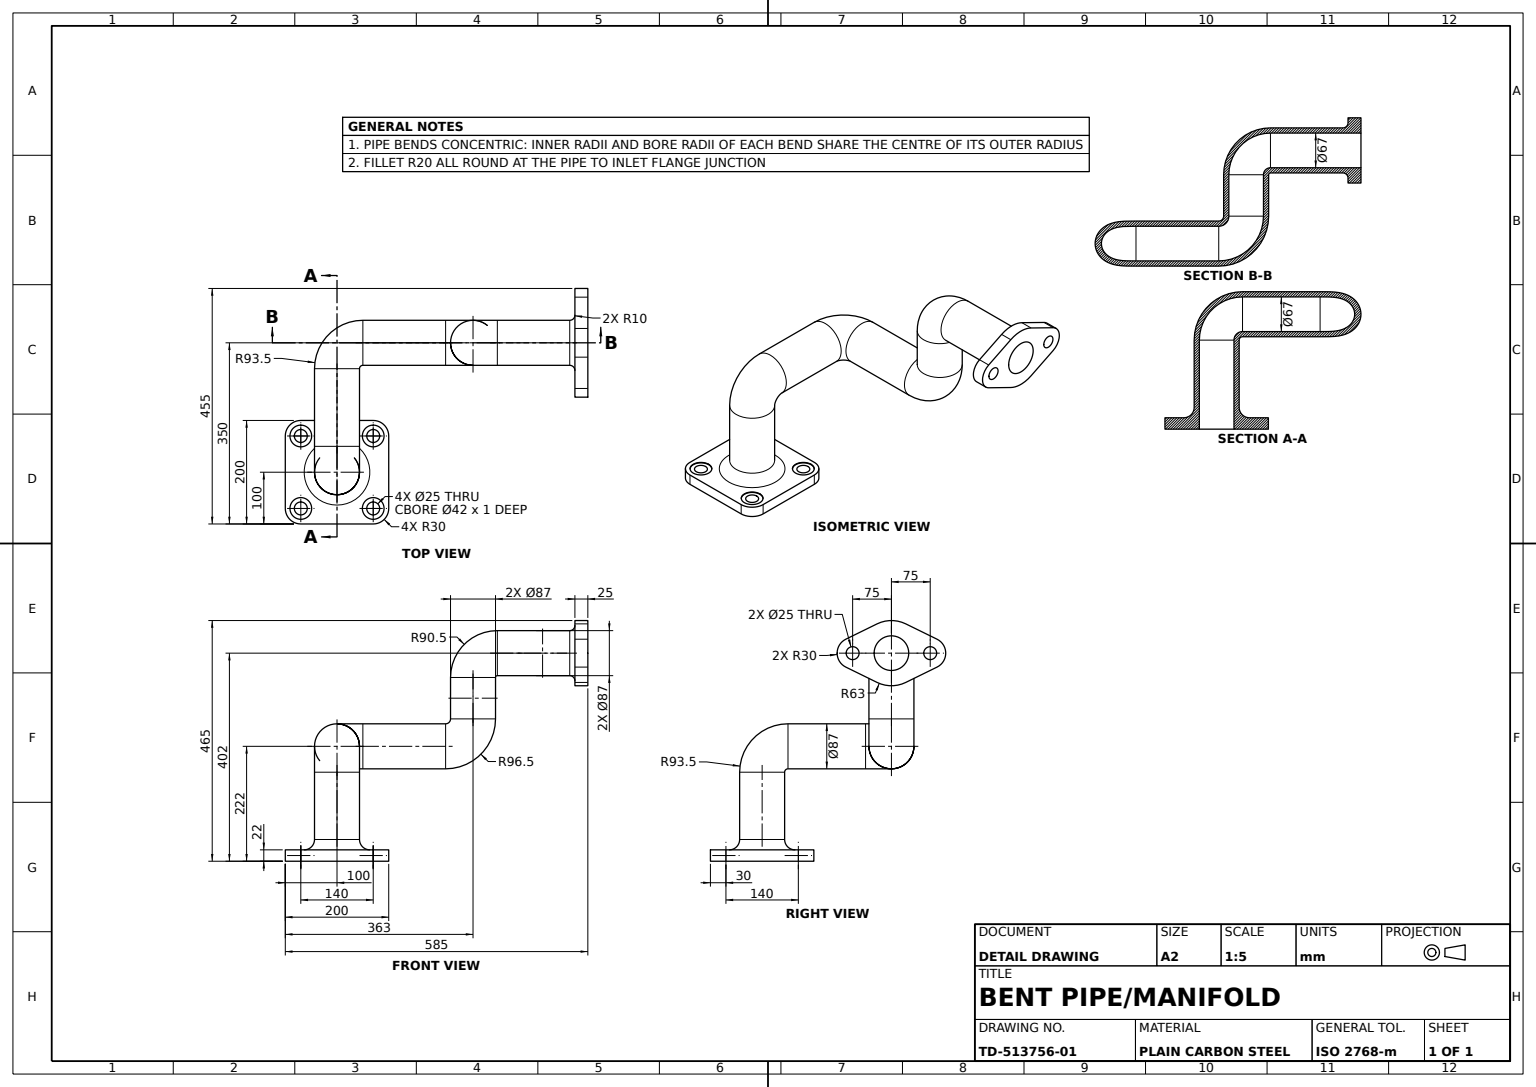
solid
v1 (70,21,-49)
v2 (70,21,-91)
e1 v1 v2 CIRCLE(AX(P(70,21,-70),D(0,1,0),D(0,0,1)),21)
e2 v2 v1 CIRCLE(AX(P(70,21,-70),D(0,1,0),D(0,0,1)),21)
v3 (70,21,-82.5)
v4 (70,21,-57.5)
e3 v3 v4 CIRCLE(AX(P(70,21,-70),D(0,1,0),D(0,0,1)),12.5)
e4 v4 v3 CIRCLE(AX(P(70,21,-70),D(0,1,0),D(0,0,1)),12.5)
face PLANE(AX(P(70,21,-70),D(0,1,0),D(0,0,1))) [e1 e2] [-e3 -e4]
v5 (485,458.57386,-277.72)
v6 (460,458.57386,-277.72)
e5 v5 v6 LINE
v7 (460,458.57386,-222.28)
e6 v6 v7 CIRCLE(AX(P(460,402,-250),D(1,0,0),D(0,0,-1)),63)
v8 (485,458.57386,-222.28)
e7 v8 v7 LINE
e8 v5 v8 CIRCLE(AX(P(485,402,-250),D(1,0,0),D(0,0,-1)),63)
face CYL(AX(P(485,402,-250),D(-1,0,0),D(0,0,1)),63) [e5 e6 -e7 -e8]
v9 (263,275,-216.5)
v10 (263,355,-216.5)
e9 v9 v10 LINE
v11 (296.5,355,-250)
e10 v10 v11 CIRCLE(AX(P(263,355,-250),D(0,1,0),D(0,0,-1)),33.5)
v12 (263,355,-283.5)
e11 v11 v12 CIRCLE(AX(P(263,355,-250),D(0,1,0),D(0,0,-1)),33.5)
v13 (263,275,-283.5)
e12 v13 v12 LINE
v14 (296.5,275,-250)
e13 v14 v13 CIRCLE(AX(P(263,275,-250),D(0,1,0),D(0,0,-1)),33.5)
e14 v9 v14 CIRCLE(AX(P(263,275,-250),D(0,1,0),D(0,0,-1)),33.5)
face CYL(AX(P(263,275,-250),D(0,1,0),D(0,0,1)),33.5) rev [e9 e10 e11 -e12 -e13 -e14]
v15 (50,222,-293.5)
v16 (50,222,-206.5)
e15 v15 v16 CIRCLE(AX(P(50,222,-250),D(1,0,0),D(0,0,-1)),43.5)
v17 (210,222,-206.5)
e16 v16 v17 LINE
v18 (210,265.5,-250)
e17 v18 v17 CIRCLE(AX(P(210,222,-250),D(1,0,0),D(0,-1,0)),43.5)
v19 (210,222,-293.5)
e18 v19 v18 CIRCLE(AX(P(210,222,-250),D(1,0,0),D(0,-1,0)),43.5)
e19 v15 v19 LINE
face CYL(AX(P(50,222,-250),D(1,0,0),D(0,0,-1)),43.5) [e15 e16 -e17 -e18 -e19]
v20 (0,42,-43.5)
v21 (0,172,-43.5)
e20 v20 v21 LINE
v22 (0,172,43.5)
e21 v22 v21 CIRCLE(AX(P(0,172,0),D(0,1,0),D(0,0,-1)),43.5)
v23 (0,42,43.5)
e22 v23 v22 LINE
e23 v23 v20 CIRCLE(AX(P(0,42,0),D(0,1,0),D(0,0,1)),43.5)
face CYL(AX(P(0,22,0),D(0,1,0),D(0,0,1)),43.5) [e20 -e21 -e22 e23]
v24 (0,0,-33.5)
v25 (0,172,-33.5)
e24 v24 v25 LINE
v26 (0,0,33.5)
e25 v26 v24 CIRCLE(AX(P(0,0,0),D(0,1,0),D(0,0,1)),33.5)
v27 (0,172,33.5)
e26 v26 v27 LINE
e27 v27 v25 CIRCLE(AX(P(0,172,0),D(0,1,0),D(0,0,1)),33.5)
face CYL(AX(P(0,-3,0),D(0,1,0),D(0,0,1)),33.5) rev [-e24 -e25 e26 e27]
v28 (70,0,-57.5)
e28 v4 v28 LINE
v29 (70,0,-82.5)
e29 v29 v28 CIRCLE(AX(P(70,0,-70),D(0,1,0),D(0,0,1)),12.5)
e30 v3 v29 LINE
face CYL(AX(P(70,22,-70),D(0,-1,0),D(0,0,-1)),12.5) rev [e3 e28 -e29 -e30]
v30 (43.5,222,-50)
v31 (43.5,222,-200)
e31 v30 v31 LINE
v32 (0,178.5,-50)
e32 v30 v32 CIRCLE(AX(P(0,222,-50),D(0,0,-1),D(-1,0,0)),43.5)
v33 (-43.5,222,-50)
e33 v32 v33 CIRCLE(AX(P(0,222,-50),D(0,0,-1),D(-1,0,0)),43.5)
v34 (-43.5,222,-200)
e34 v33 v34 LINE
e35 v31 v34 CIRCLE(AX(P(0,222,-200),D(0,0,-1),D(1,0,0)),43.5)
face CYL(AX(P(0,222,-50),D(0,0,-1),D(-1,0,0)),43.5) [-e31 e32 e33 e34 -e35]
v35 (485,402,-283.5)
v36 (485,402,-216.5)
e36 v35 v36 CIRCLE(AX(P(485,402,-250),D(1,0,0),D(0,0,-1)),33.5)
v37 (310,402,-216.5)
e37 v37 v36 LINE
v38 (310,435.5,-250)
e38 v38 v37 CIRCLE(AX(P(310,402,-250),D(1,0,0),D(0,0,-1)),33.5)
v39 (310,402,-283.5)
e39 v39 v38 CIRCLE(AX(P(310,402,-250),D(1,0,0),D(0,0,-1)),33.5)
e40 v39 v35 LINE
face CYL(AX(P(310,402,-250),D(1,0,0),D(0,0,-1)),33.5) rev [e36 -e37 -e38 -e39 e40]
v40 (100,22,-70)
v41 (100,0,-70)
e41 v40 v41 LINE
v42 (70,0,-100)
e42 v41 v42 CIRCLE(AX(P(70,0,-70),D(0,1,0),D(0,0,-1)),30)
v43 (70,22,-100)
e43 v43 v42 LINE
e44 v40 v43 CIRCLE(AX(P(70,22,-70),D(0,1,0),D(0,0,-1)),30)
face CYL(AX(P(70,22,-70),D(0,-1,0),D(0,0,-1)),30) [e41 e42 -e43 -e44]
v44 (70,21,49)
v45 (70,22,49)
e45 v44 v45 LINE
v46 (70,22,91)
e46 v45 v46 CIRCLE(AX(P(70,22,70),D(0,1,0),D(0,0,1)),21)
v47 (70,21,91)
e47 v47 v46 LINE
e48 v44 v47 CIRCLE(AX(P(70,21,70),D(0,1,0),D(0,0,1)),21)
face CYL(AX(P(70,21,70),D(0,1,0),D(0,0,1)),21) rev [e45 e46 -e47 -e48]
v48 (70,22,-49)
e49 v1 v48 LINE
v49 (70,22,-91)
e50 v48 v49 CIRCLE(AX(P(70,22,-70),D(0,1,0),D(0,0,1)),21)
e51 v2 v49 LINE
face CYL(AX(P(70,21,-70),D(0,1,0),D(0,0,1)),21) rev [-e1 e49 e50 -e51]
v50 (229.5,275,-250)
e52 v50 v9 CIRCLE(AX(P(263,275,-250),D(0,1,0),D(0,0,-1)),33.5)
v51 (210,188.5,-250)
e53 v51 v14 CIRCLE(AX(P(210,275,-250),D(0,0,1),D(1,0,0)),86.5)
v52 (210,222,-216.5)
e54 v52 v51 CIRCLE(AX(P(210,222,-250),D(1,0,0),D(0,0,-1)),33.5)
v53 (210,255.5,-250)
e55 v53 v52 CIRCLE(AX(P(210,222,-250),D(1,0,0),D(0,0,-1)),33.5)
e56 v53 v50 CIRCLE(AX(P(210,275,-250),D(0,0,1),D(1,0,0)),19.5)
face TORUS(AX(P(210,275,-250),D(0,0,1),D(1,0,0)),53,33.5) rev [e52 e14 -e53 -e54 -e55 e56]
v54 (485,345.42614,-277.72)
v55 (460,345.42614,-277.72)
e57 v54 v55 LINE
v56 (460,375.060067,-338.2)
e58 v55 v56 LINE
v57 (485,375.060067,-338.2)
e59 v57 v56 LINE
e60 v54 v57 LINE
face PLANE(AX(P(485,345.42614,-277.72),D(0,0.897997773,0.44),D(0,-0.44,0.897997773))) rev [e57 e58 -e59 -e60]
e61 v24 v26 CIRCLE(AX(P(0,0,0),D(0,1,0),D(0,0,1)),33.5)
e62 v25 v27 CIRCLE(AX(P(0,172,0),D(0,1,0),D(0,0,1)),33.5)
face CYL(AX(P(0,-3,0),D(0,1,0),D(0,0,1)),33.5) rev [-e61 e24 e62 -e26]
v58 (70,0,82.5)
v59 (70,0,57.5)
e63 v58 v59 CIRCLE(AX(P(70,0,70),D(0,1,0),D(0,0,1)),12.5)
v60 (70,21,82.5)
e64 v60 v58 LINE
v61 (70,21,57.5)
e65 v60 v61 CIRCLE(AX(P(70,21,70),D(0,1,0),D(0,0,1)),12.5)
e66 v61 v59 LINE
face CYL(AX(P(70,22,70),D(0,-1,0),D(0,0,-1)),12.5) rev [-e63 -e64 e65 e66]
e67 v34 v15 CIRCLE(AX(P(50,222,-200),D(0,-1,0),D(0,0,-1)),93.5)
e68 v34 v31 CIRCLE(AX(P(0,222,-200),D(0,0,-1),D(1,0,0)),43.5)
e69 v31 v16 CIRCLE(AX(P(50,222,-200),D(0,-1,0),D(0,0,-1)),6.5)
face TORUS(AX(P(50,222,-200),D(0,-1,0),D(0,0,-1)),50,43.5) [-e67 e68 e69 -e15]
v62 (-70,21,57.5)
v63 (-70,21,82.5)
e70 v62 v63 CIRCLE(AX(P(-70,21,70),D(0,1,0),D(0,0,1)),12.5)
e71 v63 v62 CIRCLE(AX(P(-70,21,70),D(0,1,0),D(0,0,1)),12.5)
v64 (-70,21,49)
v65 (-70,21,91)
e72 v64 v65 CIRCLE(AX(P(-70,21,70),D(0,1,0),D(0,0,1)),21)
e73 v65 v64 CIRCLE(AX(P(-70,21,70),D(0,1,0),D(0,0,1)),21)
face PLANE(AX(P(-70,21,70),D(0,1,0),D(0,0,1))) [-e70 -e71] [e72 e73]
v66 (0,22,63.5)
e74 v23 v66 CIRCLE(AX(P(0,42,63.5),D(-1,0,0),D(0,0,1)),20)
e75 v20 v23 CIRCLE(AX(P(0,42,0),D(0,1,0),D(0,0,1)),43.5)
v67 (0,22,-63.5)
e76 v20 v67 CIRCLE(AX(P(0,42,-63.5),D(1,0,0),D(0,0,-1)),20)
e77 v66 v67 CIRCLE(AX(P(0,22,0),D(0,-1,0),D(0,0,1)),63.5)
face TORUS(AX(P(0,42,0),D(0,1,0),D(0,0,1)),63.5,20) rev [-e74 -e75 e76 -e77]
v68 (-70,0,82.5)
e78 v63 v68 LINE
v69 (-70,0,57.5)
e79 v62 v69 LINE
e80 v68 v69 CIRCLE(AX(P(-70,0,70),D(0,1,0),D(0,0,1)),12.5)
face CYL(AX(P(-70,22,70),D(0,-1,0),D(0,0,-1)),12.5) rev [-e78 e71 e79 -e80]
v70 (460,428.939933,-338.2)
e81 v56 v70 CIRCLE(AX(P(460,402,-325),D(1,0,0),D(0,0,-1)),30)
v71 (485,428.939933,-338.2)
e82 v71 v70 LINE
e83 v57 v71 CIRCLE(AX(P(485,402,-325),D(1,0,0),D(0,0,-1)),30)
face CYL(AX(P(485,402,-325),D(-1,0,0),D(0,0,1)),30) [e59 e81 -e82 -e83]
v72 (485,375.060067,-161.8)
v73 (460,375.060067,-161.8)
e84 v72 v73 LINE
v74 (460,345.42614,-222.28)
e85 v73 v74 LINE
v75 (485,345.42614,-222.28)
e86 v75 v74 LINE
e87 v72 v75 LINE
face PLANE(AX(P(485,375.060067,-161.8),D(0,0.897997773,-0.44),D(0,0.44,0.897997773))) rev [e84 e85 -e86 -e87]
v76 (-70,0,100)
v77 (70,0,100)
e88 v76 v77 LINE
v78 (70,22,100)
e89 v78 v77 LINE
v79 (-70,22,100)
e90 v79 v78 LINE
e91 v79 v76 LINE
face PLANE(AX(P(-70,22,100),D(0,0,-1),D(-1,0,0))) rev [e88 -e89 -e90 e91]
e92 v16 v15 CIRCLE(AX(P(50,222,-250),D(1,0,0),D(0,0,-1)),43.5)
face TORUS(AX(P(50,222,-200),D(0,-1,0),D(0,0,-1)),50,43.5) [-e69 e35 e67 -e92]
v80 (485,402,-337.5)
v81 (460,402,-337.5)
e93 v80 v81 LINE
v82 (460,402,-312.5)
e94 v82 v81 CIRCLE(AX(P(460,402,-325),D(1,0,0),D(0,0,-1)),12.5)
v83 (485,402,-312.5)
e95 v83 v82 LINE
e96 v83 v80 CIRCLE(AX(P(485,402,-325),D(1,0,0),D(0,0,-1)),12.5)
face CYL(AX(P(485,402,-325),D(-1,0,0),D(0,0,1)),12.5) rev [e93 -e94 -e95 e96]
v84 (0,265.5,-50)
e97 v84 v30 CIRCLE(AX(P(0,222,-50),D(0,0,-1),D(-1,0,0)),43.5)
e98 v22 v84 CIRCLE(AX(P(0,172,-50),D(-1,0,0),D(0,0,1)),93.5)
e99 v21 v32 CIRCLE(AX(P(0,172,-50),D(-1,0,0),D(0,0,1)),6.5)
face TORUS(AX(P(0,172,-50),D(-1,0,0),D(0,0,1)),50,43.5) [-e32 -e97 -e98 e21 e99]
v85 (0,255.5,-50)
e100 v27 v85 CIRCLE(AX(P(0,172,-50),D(-1,0,0),D(0,0,1)),83.5)
v86 (0,188.5,-50)
e101 v25 v86 CIRCLE(AX(P(0,172,-50),D(-1,0,0),D(0,0,1)),16.5)
v87 (-33.5,222,-50)
e102 v86 v87 CIRCLE(AX(P(0,222,-50),D(0,0,-1),D(0,1,0)),33.5)
e103 v87 v85 CIRCLE(AX(P(0,222,-50),D(0,0,-1),D(0,1,0)),33.5)
face TORUS(AX(P(0,172,-50),D(-1,0,0),D(0,0,1)),50,33.5) rev [-e100 -e62 e101 e102 e103]
v88 (229.5,355,-250)
e104 v88 v38 CIRCLE(AX(P(310,355,-250),D(0,0,-1),D(-1,0,0)),80.5)
e105 v12 v88 CIRCLE(AX(P(263,355,-250),D(0,1,0),D(0,0,-1)),33.5)
v89 (310,368.5,-250)
e106 v11 v89 CIRCLE(AX(P(310,355,-250),D(0,0,-1),D(-1,0,0)),13.5)
e107 v89 v39 CIRCLE(AX(P(310,402,-250),D(1,0,0),D(0,0,-1)),33.5)
face TORUS(AX(P(310,355,-250),D(0,0,-1),D(-1,0,0)),47,33.5) rev [e39 -e104 -e105 -e11 e106 e107]
e108 v13 v50 CIRCLE(AX(P(263,275,-250),D(0,1,0),D(0,0,-1)),33.5)
v90 (210,222,-283.5)
e109 v90 v53 CIRCLE(AX(P(210,222,-250),D(1,0,0),D(0,0,-1)),33.5)
e110 v51 v90 CIRCLE(AX(P(210,222,-250),D(1,0,0),D(0,0,-1)),33.5)
face TORUS(AX(P(210,275,-250),D(0,0,1),D(1,0,0)),53,33.5) rev [e53 e13 e108 -e56 -e109 -e110]
v91 (-100,22,70)
e111 v91 v79 CIRCLE(AX(P(-70,22,70),D(0,1,0),D(0,0,1)),30)
v92 (-100,0,70)
e112 v91 v92 LINE
e113 v92 v76 CIRCLE(AX(P(-70,0,70),D(0,1,0),D(0,0,1)),30)
face CYL(AX(P(-70,22,70),D(0,-1,0),D(0,0,-1)),30) [-e111 e112 e113 -e91]
v93 (263,275,-206.5)
v94 (306.5,275,-250)
e114 v93 v94 CIRCLE(AX(P(263,275,-250),D(0,1,0),D(0,0,1)),43.5)
v95 (263,275,-293.5)
e115 v94 v95 CIRCLE(AX(P(263,275,-250),D(0,1,0),D(0,0,1)),43.5)
v96 (263,355,-293.5)
e116 v95 v96 LINE
v97 (306.5,355,-250)
e117 v97 v96 CIRCLE(AX(P(263,355,-250),D(0,1,0),D(1,0,0)),43.5)
v98 (263,355,-206.5)
e118 v98 v97 CIRCLE(AX(P(263,355,-250),D(0,1,0),D(1,0,0)),43.5)
e119 v93 v98 LINE
face CYL(AX(P(263,275,-250),D(0,1,0),D(0,0,1)),43.5) [e114 e115 e116 -e117 -e118 -e119]
v99 (485,402,-162.5)
v100 (460,402,-162.5)
e120 v99 v100 LINE
v101 (460,402,-187.5)
e121 v101 v100 CIRCLE(AX(P(460,402,-175),D(1,0,0),D(0,0,-1)),12.5)
v102 (485,402,-187.5)
e122 v102 v101 LINE
e123 v102 v99 CIRCLE(AX(P(485,402,-175),D(1,0,0),D(0,0,-1)),12.5)
face CYL(AX(P(485,402,-175),D(-1,0,0),D(0,0,1)),12.5) rev [e120 -e121 -e122 e123]
v103 (33.5,222,-50)
e124 v85 v103 CIRCLE(AX(P(0,222,-50),D(0,0,-1),D(0,1,0)),33.5)
v104 (-33.5,222,-200)
e125 v87 v104 LINE
v105 (33.5,222,-200)
e126 v104 v105 CIRCLE(AX(P(0,222,-200),D(0,0,-1),D(-1,0,0)),33.5)
e127 v103 v105 LINE
face CYL(AX(P(0,222,-50),D(0,0,-1),D(-1,0,0)),33.5) rev [-e124 -e103 e125 e126 -e127]
v106 (50,222,-216.5)
e128 v106 v52 LINE
v107 (50,222,-283.5)
e129 v107 v106 CIRCLE(AX(P(50,222,-250),D(1,0,0),D(0,0,-1)),33.5)
e130 v107 v90 LINE
face CYL(AX(P(50,222,-250),D(1,0,0),D(0,0,-1)),33.5) rev [e55 -e128 -e129 e130 e109]
e131 v106 v107 CIRCLE(AX(P(50,222,-250),D(1,0,0),D(0,0,-1)),33.5)
face CYL(AX(P(50,222,-250),D(1,0,0),D(0,0,-1)),33.5) rev [e54 e110 -e130 -e131 e128]
e132 v69 v68 CIRCLE(AX(P(-70,0,70),D(0,1,0),D(0,0,1)),12.5)
face CYL(AX(P(-70,22,70),D(0,-1,0),D(0,0,-1)),12.5) rev [e78 -e132 -e79 e70]
e133 v105 v106 CIRCLE(AX(P(50,222,-200),D(0,-1,0),D(0,0,-1)),16.5)
e134 v104 v107 CIRCLE(AX(P(50,222,-200),D(0,-1,0),D(0,0,-1)),83.5)
face TORUS(AX(P(50,222,-200),D(0,-1,0),D(0,0,-1)),50,33.5) rev [-e133 -e126 e134 e129]
v108 (-70,22,-100)
v109 (-100,22,-70)
e135 v108 v109 CIRCLE(AX(P(-70,22,-70),D(0,1,0),D(0,0,1)),30)
v110 (-70,0,-100)
e136 v108 v110 LINE
v111 (-100,0,-70)
e137 v110 v111 CIRCLE(AX(P(-70,0,-70),D(0,1,0),D(0,0,1)),30)
e138 v109 v111 LINE
face CYL(AX(P(-70,22,-70),D(0,-1,0),D(0,0,-1)),30) [-e135 e136 e137 -e138]
e139 v33 v84 CIRCLE(AX(P(0,222,-50),D(0,0,-1),D(-1,0,0)),43.5)
face CYL(AX(P(0,222,-50),D(0,0,-1),D(-1,0,0)),43.5) [e31 -e68 -e34 e139 e97]
e140 v28 v29 CIRCLE(AX(P(70,0,-70),D(0,1,0),D(0,0,1)),12.5)
face CYL(AX(P(70,22,-70),D(0,-1,0),D(0,0,-1)),12.5) rev [e30 -e140 -e28 e4]
e141 v37 v89 CIRCLE(AX(P(310,402,-250),D(1,0,0),D(0,0,-1)),33.5)
e142 v36 v35 CIRCLE(AX(P(485,402,-250),D(1,0,0),D(0,0,-1)),33.5)
face CYL(AX(P(310,402,-250),D(1,0,0),D(0,0,-1)),33.5) rev [-e40 -e107 -e141 e37 e142]
e143 v80 v83 CIRCLE(AX(P(485,402,-325),D(1,0,0),D(0,0,-1)),12.5)
e144 v81 v82 CIRCLE(AX(P(460,402,-325),D(1,0,0),D(0,0,-1)),12.5)
face CYL(AX(P(485,402,-325),D(-1,0,0),D(0,0,1)),12.5) rev [-e93 e143 e95 -e144]
v112 (450,402,-206.5)
v113 (450,402,-293.5)
e145 v112 v113 CIRCLE(AX(P(450,402,-250),D(-1,0,0),D(0,0,-1)),43.5)
v114 (460,402,-196.5)
e146 v114 v112 CIRCLE(AX(P(450,402,-196.5),D(0,1,0),D(0,0,1)),10)
v115 (460,402,-303.5)
e147 v115 v114 CIRCLE(AX(P(460,402,-250),D(1,0,0),D(0,0,-1)),53.5)
e148 v115 v113 CIRCLE(AX(P(450,402,-303.5),D(0,-1,0),D(0,0,-1)),10)
face TORUS(AX(P(450,402,-250),D(1,0,0),D(0,0,-1)),53.5,10) rev [-e145 -e146 -e147 e148]
e149 v74 v55 CIRCLE(AX(P(460,402,-250),D(1,0,0),D(0,0,-1)),63)
e150 v75 v54 CIRCLE(AX(P(485,402,-250),D(1,0,0),D(0,0,-1)),63)
face CYL(AX(P(485,402,-250),D(-1,0,0),D(0,0,1)),63) [e86 e149 -e57 -e150]
e151 v47 v44 CIRCLE(AX(P(70,21,70),D(0,1,0),D(0,0,1)),21)
e152 v61 v60 CIRCLE(AX(P(70,21,70),D(0,1,0),D(0,0,1)),12.5)
face PLANE(AX(P(70,21,70),D(0,1,0),D(0,0,1))) [e151 e48] [-e152 -e65]
v116 (-70,0,-57.5)
v117 (-70,0,-82.5)
e153 v116 v117 CIRCLE(AX(P(-70,0,-70),D(0,1,0),D(0,0,1)),12.5)
v118 (-70,21,-57.5)
e154 v118 v116 LINE
v119 (-70,21,-82.5)
e155 v118 v119 CIRCLE(AX(P(-70,21,-70),D(0,1,0),D(0,0,1)),12.5)
e156 v119 v117 LINE
face CYL(AX(P(-70,22,-70),D(0,-1,0),D(0,0,-1)),12.5) rev [-e153 -e154 e155 e156]
e157 v46 v45 CIRCLE(AX(P(70,22,70),D(0,1,0),D(0,0,1)),21)
face CYL(AX(P(70,21,70),D(0,1,0),D(0,0,1)),21) rev [e47 e157 -e45 -e151]
v120 (-70,22,49)
v121 (-70,22,91)
e158 v120 v121 CIRCLE(AX(P(-70,22,70),D(0,1,0),D(0,0,1)),21)
e159 v65 v121 LINE
e160 v64 v120 LINE
face CYL(AX(P(-70,21,70),D(0,1,0),D(0,0,1)),21) rev [e158 -e159 -e72 e160]
e161 v70 v6 LINE
e162 v71 v5 LINE
face PLANE(AX(P(485,458.57386,-277.72),D(0,-0.897997773,0.44),D(0,-0.44,-0.897997773))) rev [e82 e161 -e5 -e162]
e163 v100 v101 CIRCLE(AX(P(460,402,-175),D(1,0,0),D(0,0,-1)),12.5)
e164 v114 v115 CIRCLE(AX(P(460,402,-250),D(1,0,0),D(0,0,-1)),53.5)
v122 (460,402,-145)
e165 v122 v73 CIRCLE(AX(P(460,402,-175),D(1,0,0),D(0,0,-1)),30)
v123 (460,428.939933,-161.8)
e166 v123 v122 CIRCLE(AX(P(460,402,-175),D(1,0,0),D(0,0,-1)),30)
e167 v7 v123 LINE
face PLANE(AX(P(460,402,-175),D(1,0,0),D(0,0,-1))) rev [e121 e163] [e164 e147] [e144 e94] [-e58 -e149 -e85 -e165 -e166 -e167 -e6 -e161 -e81]
e168 v119 v118 CIRCLE(AX(P(-70,21,-70),D(0,1,0),D(0,0,1)),12.5)
e169 v117 v116 CIRCLE(AX(P(-70,0,-70),D(0,1,0),D(0,0,1)),12.5)
face CYL(AX(P(-70,22,-70),D(0,-1,0),D(0,0,-1)),12.5) rev [e168 e154 -e169 -e156]
v124 (100,0,70)
e170 v124 v41 LINE
v125 (100,22,70)
e171 v125 v40 LINE
e172 v125 v124 LINE
face PLANE(AX(P(100,22,-70),D(-1,0,0),D(0,0,1))) rev [e170 -e41 -e171 e172]
v126 (219.5,355,-250)
v127 (310,445.5,-250)
e173 v126 v127 CIRCLE(AX(P(310,355,-250),D(0,0,-1),D(-1,0,0)),90.5)
e174 v126 v98 CIRCLE(AX(P(263,355,-250),D(0,1,0),D(1,0,0)),43.5)
v128 (310,358.5,-250)
e175 v97 v128 CIRCLE(AX(P(310,355,-250),D(0,0,-1),D(-1,0,0)),3.5)
v129 (310,402,-206.5)
e176 v129 v128 CIRCLE(AX(P(310,402,-250),D(1,0,0),D(0,0,-1)),43.5)
e177 v127 v129 CIRCLE(AX(P(310,402,-250),D(1,0,0),D(0,0,-1)),43.5)
face TORUS(AX(P(310,355,-250),D(0,0,-1),D(-1,0,0)),47,43.5) [-e173 e174 e118 e175 -e176 -e177]
e178 v113 v112 CIRCLE(AX(P(450,402,-250),D(-1,0,0),D(0,0,-1)),43.5)
face TORUS(AX(P(450,402,-250),D(1,0,0),D(0,0,-1)),53.5,10) rev [-e164 e146 -e178 -e148]
v130 (485,402,-145)
e179 v130 v122 LINE
e180 v130 v72 CIRCLE(AX(P(485,402,-175),D(1,0,0),D(0,0,-1)),30)
face CYL(AX(P(485,402,-175),D(-1,0,0),D(0,0,1)),30) [e179 e165 -e84 -e180]
e181 v77 v124 CIRCLE(AX(P(70,0,70),D(0,1,0),D(0,0,1)),30)
e182 v78 v125 CIRCLE(AX(P(70,22,70),D(0,1,0),D(0,0,1)),30)
face CYL(AX(P(70,22,70),D(0,-1,0),D(0,0,-1)),30) [e181 -e172 -e182 e89]
e183 v59 v58 CIRCLE(AX(P(70,0,70),D(0,1,0),D(0,0,1)),12.5)
face CYL(AX(P(70,22,70),D(0,-1,0),D(0,0,-1)),12.5) rev [e64 -e183 -e66 e152]
e184 v103 v86 CIRCLE(AX(P(0,222,-50),D(0,0,-1),D(0,1,0)),33.5)
face TORUS(AX(P(0,172,-50),D(-1,0,0),D(0,0,1)),50,33.5) rev [-e101 -e27 e100 e124 e184]
e185 v129 v112 LINE
v131 (310,402,-293.5)
e186 v131 v113 LINE
e187 v131 v127 CIRCLE(AX(P(310,402,-250),D(1,0,0),D(0,0,-1)),43.5)
face CYL(AX(P(310,402,-250),D(1,0,0),D(0,0,-1)),43.5) [e185 e145 -e186 e187 e177]
e188 v21 v22 CIRCLE(AX(P(0,172,0),D(0,1,0),D(0,0,-1)),43.5)
face TORUS(AX(P(0,172,-50),D(-1,0,0),D(0,0,1)),50,43.5) [-e33 -e99 e188 e98 -e139]
e189 v111 v92 LINE
e190 v42 v110 LINE
face PLANE(AX(P(70,0,70),D(0,1,0),D(0,0,1))) rev [e63 e183] [e61 e25] [e169 e153] [e29 e140] [e132 e80] [-e181 -e88 -e113 -e189 -e137 -e190 -e42 -e170]
v132 (-70,22,-91)
v133 (-70,22,-49)
e191 v132 v133 CIRCLE(AX(P(-70,22,-70),D(0,1,0),D(0,0,1)),21)
v134 (-70,21,-49)
e192 v134 v133 LINE
v135 (-70,21,-91)
e193 v135 v134 CIRCLE(AX(P(-70,21,-70),D(0,1,0),D(0,0,1)),21)
e194 v135 v132 LINE
face CYL(AX(P(-70,21,-70),D(0,1,0),D(0,0,1)),21) rev [e191 -e192 -e193 e194]
e195 v96 v126 CIRCLE(AX(P(263,355,-250),D(0,1,0),D(1,0,0)),43.5)
v136 (219.5,275,-250)
e196 v95 v136 CIRCLE(AX(P(263,275,-250),D(0,1,0),D(0,0,1)),43.5)
e197 v136 v93 CIRCLE(AX(P(263,275,-250),D(0,1,0),D(0,0,1)),43.5)
face CYL(AX(P(263,275,-250),D(0,1,0),D(0,0,1)),43.5) [-e195 -e116 e196 e197 e119 -e174]
v137 (485,428.939933,-161.8)
e198 v8 v137 LINE
e199 v137 v123 LINE
face PLANE(AX(P(485,458.57386,-222.28),D(0,-0.897997773,-0.44),D(0,0.44,-0.897997773))) rev [-e198 e7 e167 -e199]
e200 v105 v104 CIRCLE(AX(P(0,222,-200),D(0,0,-1),D(-1,0,0)),33.5)
face CYL(AX(P(0,222,-50),D(0,0,-1),D(-1,0,0)),33.5) rev [e127 e200 -e125 -e102 -e184]
e201 v99 v102 CIRCLE(AX(P(485,402,-175),D(1,0,0),D(0,0,-1)),12.5)
face CYL(AX(P(485,402,-175),D(-1,0,0),D(0,0,1)),12.5) rev [-e120 e201 e122 -e163]
e202 v49 v48 CIRCLE(AX(P(70,22,-70),D(0,1,0),D(0,0,1)),21)
face CYL(AX(P(70,21,-70),D(0,1,0),D(0,0,1)),21) rev [e51 e202 -e49 -e2]
e203 v43 v108 LINE
face PLANE(AX(P(-70,22,-100),D(0,0,1),D(1,0,0))) rev [e190 -e136 -e203 e43]
e204 v133 v132 CIRCLE(AX(P(-70,22,-70),D(0,1,0),D(0,0,1)),21)
e205 v67 v66 CIRCLE(AX(P(0,22,0),D(0,-1,0),D(0,0,1)),63.5)
e206 v109 v91 LINE
e207 v121 v120 CIRCLE(AX(P(-70,22,70),D(0,1,0),D(0,0,1)),21)
face PLANE(AX(P(70,22,70),D(0,1,0),D(0,0,1))) [-e204 -e191] [e77 e205] [e203 e135 e206 e111 e90 e182 e171 e44] [-e157 -e46] [-e207 -e158] [-e202 -e50]
v138 (210,178.5,-250)
e208 v17 v138 CIRCLE(AX(P(210,222,-250),D(1,0,0),D(0,-1,0)),43.5)
e209 v138 v19 CIRCLE(AX(P(210,222,-250),D(1,0,0),D(0,-1,0)),43.5)
face CYL(AX(P(50,222,-250),D(1,0,0),D(0,0,-1)),43.5) [-e208 -e16 e92 e19 -e209]
e210 v128 v131 CIRCLE(AX(P(310,402,-250),D(1,0,0),D(0,0,-1)),43.5)
face TORUS(AX(P(310,355,-250),D(0,0,-1),D(-1,0,0)),47,43.5) [-e210 -e175 e117 e195 e173 -e187]
face CYL(AX(P(0,22,0),D(0,1,0),D(0,0,1)),43.5) [e75 e22 -e188 -e20]
e211 v18 v136 CIRCLE(AX(P(210,275,-250),D(0,0,1),D(1,0,0)),9.5)
e212 v138 v94 CIRCLE(AX(P(210,275,-250),D(0,0,1),D(1,0,0)),96.5)
face TORUS(AX(P(210,275,-250),D(0,0,1),D(1,0,0)),53,43.5) [e209 e18 e211 -e196 -e115 -e212]
e213 v88 v10 CIRCLE(AX(P(263,355,-250),D(0,1,0),D(0,0,-1)),33.5)
face CYL(AX(P(263,275,-250),D(0,1,0),D(0,0,1)),33.5) rev [e213 -e9 -e52 -e108 e12 e105]
face TORUS(AX(P(310,355,-250),D(0,0,-1),D(-1,0,0)),47,33.5) rev [e104 e38 e141 -e106 -e10 -e213]
e214 v134 v135 CIRCLE(AX(P(-70,21,-70),D(0,1,0),D(0,0,1)),21)
face PLANE(AX(P(-70,21,-70),D(0,1,0),D(0,0,1))) [e214 e193] [-e155 -e168]
face CYL(AX(P(-70,21,-70),D(0,1,0),D(0,0,1)),21) rev [e192 e204 -e194 -e214]
face TORUS(AX(P(0,42,0),D(0,1,0),D(0,0,1)),63.5,20) rev [e74 -e205 -e76 -e23]
face TORUS(AX(P(210,275,-250),D(0,0,1),D(1,0,0)),53,43.5) [e208 e212 -e114 -e197 -e211 e17]
face PLANE(AX(P(-100,22,-70),D(1,0,0),D(0,0,-1))) rev [e189 -e112 -e206 e138]
face CYL(AX(P(310,402,-250),D(1,0,0),D(0,0,-1)),43.5) [e178 -e185 e176 e210 e186]
face CYL(AX(P(-70,21,70),D(0,1,0),D(0,0,1)),21) rev [-e73 e159 e207 -e160]
face TORUS(AX(P(50,222,-200),D(0,-1,0),D(0,0,-1)),50,33.5) rev [e131 -e134 -e200 e133]
e215 v137 v130 CIRCLE(AX(P(485,402,-175),D(1,0,0),D(0,0,-1)),30)
face CYL(AX(P(485,402,-175),D(-1,0,0),D(0,0,1)),30) [-e179 -e215 e199 e166]
face PLANE(AX(P(485,402,-175),D(1,0,0),D(0,0,-1))) [-e142 -e36] [-e96 -e143] [-e123 -e201] [e8 e198 e215 e180 e87 e150 e60 e83 e162]
